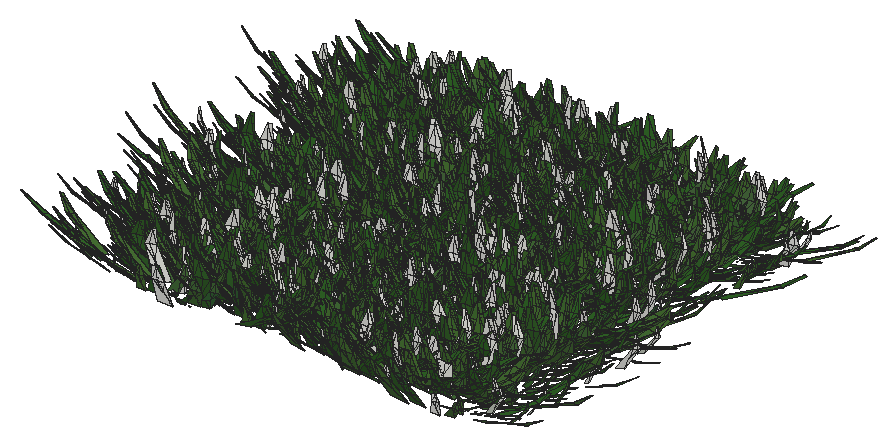
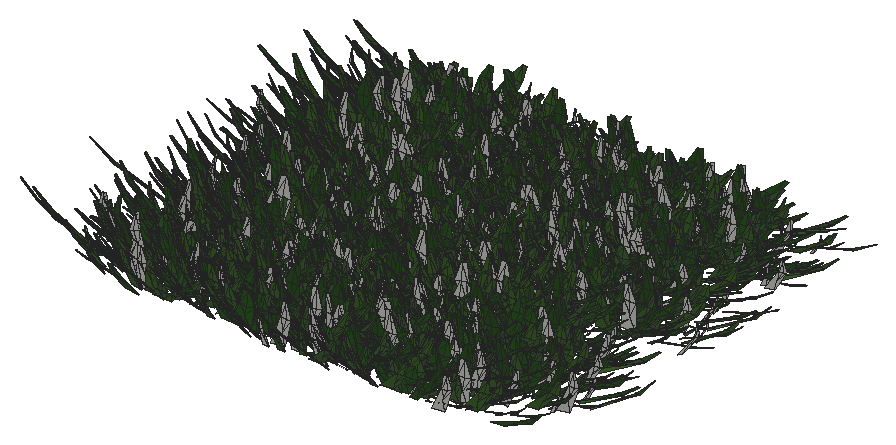
# SketchUp Ruby script. Lengths in inches.
U = 1.inch
M = Sketchup.active_model
def pt(a) = Geom::Point3d.new(a.map { |v| v * U })
def face(e, loops, mat)
  f = e.add_face(loops[0].map { |a| pt(a) })
  loops[1..].each { |l| e.add_face(l.map { |a| pt(a) }).erase! }
  f.material = f.back_material = mat if mat
  f
end
# faces: each face lists its corners as indices into pts; further lists are holes
def faces(e, pts, list, mat = nil) = list.each { |f| face(e, (f[0].is_a?(Array) ? f : [f]).map { |l| l.map { |i| pts[i] } }, mat) }
# xy, xz, yz: faces in a plane at the given z, y or x. An outline is a flat list of corners, or four numbers for a rectangle; further outlines are holes
def ring(l) = l.size == 4 ? [[l[0], l[1]], [l[2], l[1]], [l[2], l[3]], [l[0], l[3]]] : l.each_slice(2).to_a
def flat(e, list, mat, &to3) = list.each { |f| face(e, (f[0].is_a?(Array) ? f : [f]).map { |l| ring(l).map { |u, v| to3.(u, v) } }, mat) }
def xy(e, z, list, mat = nil) = flat(e, list, mat) { |x, y| [x, y, z] }
def xz(e, y, list, mat = nil) = flat(e, list, mat) { |x, z| [x, y, z] }
def yz(e, x, list, mat = nil) = flat(e, list, mat) { |y, z| [x, y, z] }
def lines(e, pts, list) = list.each { |a, b| e.add_line(pt(pts[a]), pt(pts[b])) }
# prism: a flat outline (further loops are holes) pulled along v
def prism(e, loops, v, mat = nil)
  f = face(e, loops, mat); d = Geom::Vector3d.new(v.map { |x| x * U })
  f.pushpull(f.normal.samedirection?(d) ? d.length : -d.length)
end
def box(e, o, s, mat = nil) = prism(e, [[o, [o[0] + s[0], o[1], o[2]], [o[0] + s[0], o[1] + s[1], o[2]], [o[0], o[1] + s[1], o[2]]]], [0, 0, s[2]], mat)
def at(x, y, z, deg = 0) = Geom::Transformation.translation(pt([x, y, z])) * Geom::Transformation.rotation(ORIGIN, Z_AXIS, deg.degrees)
def axes(o, x, y, z) = Geom::Transformation.new([*x, 0, *y, 0, *z, 0, *pt(o).to_a, 1])
def part(name) = M.definitions.add(name)
# library, detail: a bought-in or finely detailed component or shape, given as its bounding box
def library(name, o, s) = part(name).tap { |d| box(d.entities, o, s) }
def detail(e, o, s) = box(e.add_group.entities, o, s)
def put(e, d, t, mat = nil) = e.add_instance(d, t).tap { |i| i.material = mat if mat }
def group(e, t, mat = nil) = e.add_group.tap { |g| g.transformation = t; g.material = mat if mat }.entities
root = M.entities
M.materials.add("Material10").color = [48, 100, 38]
M.materials.add("Material3").color = [68, 110, 58]
M.materials.add("Material4").color = [48, 90, 38]
M.materials.add("Material5").color = [68, 110, 48]
M.materials.add("Material6").color = [48, 90, 48]
M.materials.add("Material7").color = [58, 110, 58]
M.materials.add("Material8").color = [58, 90, 38]
M.materials.add("Material9").color = [68, 100, 58]
c1 = part("grass00")
p = [[-0.6875,0.15,0],[-0.56,0.08,5.52],[-0.04,0.03,2.76],[0.48,-0.02,0],[0.35,-0.02,5.52],[-0.1,-0.14,5.52],
  [-0.12,0.65,8.37],[-0.42,0.65,8.37]]
faces(c1.entities,p,[[0,1,2,3],[3,2,4],[1,5,2],[5,4,2],[1,6,5],[4,5,6],[7,6,1]])
c2 = part("Group16\#1")
put(c2.entities,c1,axes([1.44,-0.61,-0.01],[0.05352,0.12609,0],[-0.10704,0.04543,0.07239],[0.06664,-0.02828,0.11628]),"Material6")
put(c2.entities,c1,axes([0.76,-0.15,-0.01],[0.04676,0.24062,0],[-0.23162,0.04501,0.06642],[0.0652,-0.01267,0.23595]),"Material3")
put(c2.entities,c1,axes([0.79,0.01,-0.01],[-0.00606,0.34651,0],[-0.34381,-0.00602,0.0432],[0.04319,0.00076,0.34386]))
put(c2.entities,c1,axes([1,0.23,-0.01],[-0.07192,0.31144,0],[-0.28722,-0.06632,0.1236],[0.12043,0.02781,0.29478]),"Material5")
put(c2.entities,c1,axes([1.66,0.77,-0.01],[-0.13828,0.29651,0],[-0.21551,-0.1005,0.22471],[0.20365,0.09498,0.23779]),"Material10")
put(c2.entities,c1,axes([0.6875,0.52,-0.01],[-0.18126,0.24051,0],[-0.22746,-0.17142,0.09788],[0.07817,0.05891,0.28481]),"Material5")
put(c2.entities,c1,axes([0.68,0.78,-0.01],[-0.215,0.18688,0],[-0.12385,-0.14248,0.21334],[0.13995,0.16101,0.18878]),"Material3")
put(c2.entities,c1,axes([0.56,1,-0.01],[-0.13756,0.07624,0],[-0.06159,-0.11112,0.0927],[0.04494,0.08108,0.12705]),"Material5")
put(c2.entities,c1,axes([0.2,0.64,-0.01],[-0.23729,0.07254,0],[-0.05711,-0.18681,0.153],[0.04473,0.14632,0.19535]),"Material10")
put(c2.entities,c1,axes([0.0625,0.72,-0.01],[-0.28874,0.02525,0],[-0.02179,-0.24916,0.14647],[0.01276,0.14591,0.25012]),"Material3")
put(c2.entities,c1,axes([-0.08,0.62,-0.01],[-0.34089,-0.04187,0],[0.03255,-0.26504,0.216],[-0.02633,0.21439,0.26703]),"Material10")
put(c2.entities,c1,axes([-0.34,0.98,-0.01],[-0.14314,-0.0493,0],[0.04397,-0.12769,0.06843],[-0.02228,0.0647,0.13505]),"Material10")
put(c2.entities,c1,axes([-0.87,1.45,-0.01],[-0.23488,-0.14114,0],[0.13761,-0.22901,0.06087],[-0.03135,0.05217,0.26717]))
put(c2.entities,c1,axes([-0.72,0.77,-0.01],[-0.14208,-0.13251,0],[0.07209,-0.0773,0.16301],[-0.11118,0.11922,0.1057]),"Material10")
put(c2.entities,c1,axes([-0.62,0.43,-0.01],[-0.14845,-0.21203,0],[0.18654,-0.13061,0.12304],[-0.10079,0.07057,0.22772]),"Material3")
put(c2.entities,c1,axes([-0.68,0.29,-0.01],[-0.13639,-0.32136,0],[0.31723,-0.13464,0.05579],[-0.05136,0.0218,0.34462]),"Material4")
put(c2.entities,c1,axes([-0.64,0.125,-0.01],[-0.0458,-0.23569,0],[0.22124,-0.043,0.08276],[-0.08124,0.01579,0.22538]),"Material7")
put(c2.entities,c1,axes([-1.6,-0.03,-0.01],[0.00576,-0.32897,0],[0.27526,0.00482,0.18018],[-0.18015,-0.00315,0.2753]),"Material5")
put(c2.entities,c1,axes([-1.36,-0.31,-0.01],[0.05718,-0.24765,0],[0.18172,0.04196,0.17267],[-0.16825,-0.03885,0.1865]),"Material10")
put(c2.entities,c1,axes([-1.54,-0.72,-0.01],[0.06537,-0.14017,0],[0.13555,0.06321,0.03939],[-0.0357,-0.01665,0.14956]))
put(c2.entities,c1,axes([-1.19,-0.9,-0.01],[0.09597,-0.12735,0],[0.11214,0.08451,0.07557],[-0.06035,-0.04548,0.14042]),"Material9")
put(c2.entities,c1,axes([-0.47,-0.54,-0.01],[0.11588,-0.10072,0],[0.0618,0.0711,0.12124],[-0.07953,-0.0915,0.0942]))
put(c2.entities,c1,axes([-0.47,-0.84,-0.01],[0.11927,-0.0661,0],[0.06603,0.11913,0.00646],[-0.00313,-0.00565,0.13621]),"Material5")
put(c2.entities,c1,axes([-0.38,-1.24,-0.01],[0.28037,-0.08571,0],[0.0618,0.20215,0.20315],[-0.05939,-0.19428,0.21139]),"Material9")
put(c2.entities,c1,axes([-0.06,-0.66,-0.01],[0.22719,-0.01987,0],[0.01247,0.14255,0.17758],[-0.01547,-0.17691,0.1431]),"Material8")
put(c2.entities,c1,axes([0.11,-0.89,-0.01],[0.14882,0.01828,0],[-0.01058,0.08611,0.12229],[0.01491,-0.12138,0.08676]),"Material6")
put(c2.entities,c1,axes([0.25,-0.72,-0.01],[0.20481,0.07053,0],[-0.06206,0.18022,0.10291],[0.03351,-0.0973,0.1906]),"Material6")
put(c2.entities,c1,axes([0.85,-1.42,-0.01],[0.16481,0.09904,0],[-0.09472,0.15762,0.05616],[0.02893,-0.04814,0.18389]),"Material5")
put(c2.entities,c1,axes([1.01,-1.09,-0.01],[0.21858,0.20385,0],[-0.17495,0.1876,0.15339],[0.10462,-0.11218,0.25652]),"Material10")
put(c2.entities,c1,axes([1.01,-0.71,-0.01],[0.08733,0.12473,0],[-0.06445,0.04512,0.13037],[0.1068,-0.07477,0.07867]),"Material6")
c3 = part("Group15\#1")
put(c3.entities,c2,at(0,0,0))
c4 = part("3darcstudiotree_grass00\#1")
put(c4.entities,c3,at(0,0,0))
put(root,c4,axes([159.13,10.51,7.6],[2.53298,-0.99579,0],[3.28482,0.52222,-0.04064],[0.20675,0.03287,1.46692]))
put(root,c4,axes([159.22,37.4375,7.6],[2.73989,-0.60489,0],[2.55091,0.72216,-0.01409],[0.06366,0.01802,1.64399]))
put(root,c4,axes([159.47,17.03,7.6],[2.49365,-0.78367,0],[3.24543,0.64544,-0.01848],[0.08233,0.01637,1.47553]))
put(root,c4,axes([158.3,36.26,7.6],[4.4609,0.40125,0],[-1.29285,0.89834,-0.01256],[-0.03244,0.02254,1.82155]))
put(root,c4,axes([158.47,24.0625,7.6],[2.4643,0.83625,0],[-3.57537,0.6585,-0.0323],[-0.14016,0.02581,1.496]))
put(root,c4,axes([159.16,32.27,7.6],[-1.53289,0.94847,0],[-3.89243,-0.39318,-0.02451],[-0.14378,-0.01452,1.66036]))
put(root,c4,axes([158.6,11.21,7.6],[3.75653,0.68918,0],[-2.16074,0.73611,-0.01519],[-0.05314,0.0181,1.34969]))
put(root,c4,axes([159.65,8.5625,7.6],[-1.332,1.0855,0],[-3.68359,-0.2825,-0.03727],[-0.23368,-0.01792,1.57911]))
put(root,c4,axes([158.96,20.36,7.6],[4.4023,0.31445,0],[-1.15221,1.00818,-0.01128],[-0.01903,0.01665,1.61003]))
put(root,c4,axes([159.3125,22.22,7.6],[4.69374,-0.30667,0],[0.9938,0.95067,-0.02428],[0.04983,0.04767,1.99391]))
put(root,c4,axes([159.65,34.32,7.6],[3.84654,0.1622,0],[-0.71389,1.05813,-0.03005],[-0.02875,0.04262,1.54341]))
put(root,c4,axes([160.2,5.28,7.6],[3.63097,-0.44195,0],[1.99155,1.02264,-0.02466],[0.05688,0.02921,1.49812]))
put(root,c4,axes([160.53,29.87,7.6],[-0.92615,0.92755,0],[-3.93926,-0.24583,-0.00012],[-0.00062,-0.00004,1.39497]))
put(root,c4,axes([160.89,40.6,7.6],[-1.66158,1.03755,0],[-3.61607,-0.36193,-0.01826],[-0.10251,-0.01026,1.47196]))
put(root,c4,axes([161.29,14.89,7.6],[3.53421,-0.66797,0],[2.63257,0.87056,-0.04167],[0.17144,0.05669,1.86151]))
put(root,c4,axes([162.89,12.95,7.6],[-3.75679,-0.65225,0],[2.19929,-0.79171,-0.00375],[0.0162,-0.00583,1.82358]))
put(root,c4,axes([162.96,8.51,7.6],[-3.06353,-0.57111,0],[2.62826,-0.88115,-0.00029],[0.00107,-0.00036,1.69542]))
put(root,c4,axes([161.18,31.73,7.6],[4.12285,0.65297,0],[-2.36966,0.93513,-0.03414],[-0.094,0.03709,1.42377]))
put(root,c4,axes([163.05,18.05,7.6],[-4.09682,0.49001,0],[-2.11354,-1.10442,-0.05113],[-0.09658,-0.05047,1.33965]))
put(root,c4,axes([163.35,33.23,7.6],[3.22149,-0.77184,0],[3.4883,0.90996,-0.03986],[0.14566,0.038,1.66404]))
put(root,c4,axes([163.88,5.03,7.6],[-3.99831,0.66373,0],[-2.79382,-1.05187,-0.05111],[-0.13772,-0.05185,1.53759]))
put(root,c4,axes([163.84,23.63,7.6],[-2.34879,0.82115,0],[-3.6953,-0.66061,-0.05929],[-0.24052,-0.043,1.41608]))
put(root,c4,axes([162.93,11.58,7.6],[2.86716,0.8976,0],[-2.85293,0.56956,-0.01421],[-0.0686,0.0137,1.40932]))
put(root,c4,axes([164.88,34.3,7.6],[-0.2584,-1.18473,0],[3.63618,-0.04957,-0.01049],[0.06761,-0.00092,1.4693]))
put(root,c4,axes([165.875,35.68,7.6],[-2.94405,-0.59903,0],[3.18153,-0.97726,-0.04334],[0.11663,-0.03583,1.34295]))
put(root,c4,axes([165.14,31.64,7.6],[2.52087,-0.77867,0],[3.74489,0.75773,-0.0352],[0.16916,0.03423,1.86157]))
put(root,c4,axes([166.21,29.5625,7.6],[-4.25461,-0.72001,0],[2.67413,-0.98761,-0.04034],[0.12328,-0.04553,1.62559]))
put(root,c4,axes([163.93,16.3,7.6],[4.6579,0.46394,0],[-1.71341,1.07515,-0.01606],[-0.03179,0.01995,1.54782]))
put(root,c4,axes([164.26,28.29,7.6],[1.00242,0.87576,0],[-4.78791,0.34253,-0.02742],[-0.16399,0.01173,1.93645]))
put(root,c4,axes([164.54,21.99,7.6],[-0.10924,0.93543,0],[-4.47278,-0.03265,-0.00454],[-0.02701,-0.0002,1.66362]))
put(root,c4,axes([166.71,20.63,7.6],[-1.41075,-1.20737,0],[3.77402,-0.27561,-0.03009],[0.20256,-0.01479,1.72353]))
put(root,c4,axes([165.51,42.17,7.6],[4.18656,0.30844,0],[-1.02812,0.87218,-0.026],[-0.05159,0.04376,1.59572]))
put(root,c4,axes([167.1875,39.94,7.6],[1.76759,-1.11088,0],[4.77436,0.4748,-0.04298],[0.2101,0.02089,1.68954]))
put(root,c4,axes([165.72,38.26,7.6],[4.47643,0.35496,0],[-1.36564,1.07638,-0.00141],[-0.00295,0.00232,1.95289]))
put(root,c4,axes([166.25,7.31,7.6],[0.44827,0.96887,0],[-3.98401,0.1152,-0.04522],[-0.2884,0.00834,1.60941]))
put(root,c4,axes([166.69,10.33,7.6],[-3.25483,0.8021,0],[-3.45367,-0.87591,-0.01243],[-0.05011,-0.01271,1.76595]))
put(root,c4,axes([166.71,36.98,7.6],[4.42338,-0.02191,0],[0.0799,1.00813,-0.01855],[0.00282,0.03561,1.93628]))
put(root,c4,axes([166.8,14.59,7.6],[1.52901,1.13008,0],[-3.97535,0.33617,-0.04556],[-0.25323,0.02141,1.53888]))
put(root,c4,axes([167.35,18.53,7.6],[4.69014,-0.44413,0],[1.55704,1.02768,-0.01068],[0.01805,0.01192,1.31138]))
put(root,c4,axes([167.31,27.18,7.6],[3.67709,0.37589,0],[-1.7272,1.05602,-0.03911],[-0.07805,0.04772,1.50402]))
put(root,c4,axes([169.42,21.05,7.6],[-2.16175,-1.00389,0],[3.8462,-0.51764,-0.02018],[0.12706,-0.0171,1.95264]))
put(root,c4,axes([169.36,31.17,7.6],[-2.62411,-0.67542,0],[2.85989,-0.69444,-0.02073],[0.09247,-0.02245,1.5494]))
put(root,c4,axes([167.22,25.11,7.6],[2.20682,1.15051,0],[-3.88825,0.46614,-0.00104],[-0.00548,0.00066,1.58037]))
put(root,c4,axes([169.95,29.43,7.6],[-3.73719,-0.68313,0],[2.19401,-0.75016,-0.03203],[0.15881,-0.0543,1.95145]))
put(root,c4,axes([169.06,5.71,7.6],[3.66888,-0.3039,0],[1.21402,0.91602,-0.03222],[0.07511,0.05667,1.78787]))
put(root,c4,axes([169.76,41.57,7.6],[2.44539,-0.83578,0],[3.06971,0.56135,-0.02877],[0.14565,0.02664,1.49076]))
put(root,c4,axes([171.36,26.94,7.6],[-2.07648,-1.05782,0],[4.05072,-0.49696,-0.01008],[0.05023,-0.00616,1.566]))
put(root,c4,axes([169.62,8.06,7.6],[0.11038,0.92839,0],[-4.43569,0.03296,-0.05613],[-0.30865,0.00229,1.5259]))
put(root,c4,axes([170.4,23.125,7.6],[3.30121,-0.61217,0],[2.52484,0.85098,-0.02804],[0.09819,0.03309,1.55696]))
put(root,c4,axes([169.56,7.46,7.6],[2.77049,0.67206,0],[-2.57835,0.66431,-0.00683],[-0.0359,0.00925,1.74693]))
put(root,c4,axes([171.22,38.9375,7.6],[-4.82674,0.25422,0],[-0.88565,-1.05095,-0.00142],[-0.00177,-0.0021,1.63114]))
put(root,c4,axes([171.51,24.73,7.6],[-4.23216,-0.4101,0],[1.59131,-1.02639,-0.05586],[0.14093,-0.0909,1.92103]))
put(root,c4,axes([171.66,13.95,7.6],[0.04875,-0.97285,0],[3.90965,0.01225,-0.00992],[0.05364,0.00017,1.32167]))
put(root,c4,axes([171.35,40.41,7.6],[-4.10192,0.74973,0],[-2.75988,-0.94373,-0.03994],[-0.15914,-0.05442,1.97331]))
put(root,c4,axes([170.21,35.1875,7.6],[5.03069,0.15304,0],[-0.59852,1.22962,-0.0359],[-0.02633,0.0541,1.88046]))
put(root,c4,axes([171.68,32.1875,7.6],[1.61139,-0.92057,0],[3.30633,0.36172,-0.00213],[0.01129,0.00123,1.30651]))
put(root,c4,axes([172.91,9.63,7.6],[-2.89418,-0.78817,0],[3.81113,-0.87466,-0.02326],[0.09657,-0.02216,1.82249]))
put(root,c4,axes([172.31,11.86,7.6],[1.38566,-1.0009,0],[3.42279,0.29616,-0.00044],[0.00245,0.00021,1.32507]))
put(root,c4,axes([172.875,18.86,7.6],[-4.53149,-0.15613,0],[0.63638,-1.15439,-0.00876],[0.00543,-0.00985,1.32289]))
put(root,c4,axes([171.83,34.23,7.6],[-3.16538,1.0009,0],[-3.18179,-0.62891,-0.0043],[-0.02493,-0.00493,1.8735]))
put(root,c4,axes([170.84,28.53,7.6],[2.46284,0.96083,0],[-4.30352,0.68944,-0.02786],[-0.14516,0.02326,1.9768]))
put(root,c4,axes([171.89,12.7,7.6],[3.73009,0.22757,0],[-0.89297,0.9148,-0.01459],[-0.0258,0.02643,1.75568]))
put(root,c4,axes([172.13,37.66,7.6],[5.05197,-0.08472,0],[0.33414,1.24538,-0.00473],[0.00152,0.00566,1.49489]))
put(root,c4,axes([172.04,16.05,7.6],[3.94341,0.43089,0],[-1.69112,0.9673,-0.01451],[-0.03524,0.02016,1.59989]))
put(root,c4,axes([173.25,17.83,7.6],[-1.02018,1.09305,0],[-3.99403,-0.23299,-0.02125],[-0.10851,-0.00633,1.34411]))
put(root,c4,axes([173.11,21.67,7.6],[1.6819,1.04129,0],[-4.31148,0.43525,-0.05886],[-0.25156,0.0254,1.33951]))
put(root,c4,axes([175.58,17.4375,7.6],[-2.51512,-0.77135,0],[3.2397,-0.66023,-0.00371],[0.01648,-0.00336,1.4993]))
put(root,c4,axes([175.5,42,7.6],[-2.73008,-0.65952,0],[3.11842,-0.80679,-0.03177],[0.14282,-0.03695,1.8145]))
put(root,c4,axes([175.29,21.77,7.6],[-3.14493,1.01166,0],[-3.08712,-0.59981,-0.03149],[-0.13615,-0.02645,1.33797]))
put(root,c4,axes([175.24,15.97,7.6],[-3.00004,0.96775,0],[-4.04392,-0.78352,-0.03455],[-0.13505,-0.02617,1.58129]))
put(root,c4,axes([176.8125,35.56,7.6],[-3.06002,-0.4895,0],[1.9457,-0.7602,-0.02395],[0.07981,-0.03118,1.39534]))
put(root,c4,axes([175.51,9.49,7.6],[4.73916,-0.2961,0],[1.22977,1.23018,-0.03338],[0.03516,0.03517,1.37691]))
put(root,c4,axes([175.81,27.67,7.6],[3.7155,-0.16397,0],[0.83101,1.17689,-0.03701],[0.04274,0.06052,1.98432]))
put(root,c4,axes([175.75,33.74,7.6],[1.11685,0.86772,0],[-3.58583,0.28846,-0.0339],[-0.24805,0.01995,1.80984]))
put(root,c4,axes([176.24,14.33,7.6],[3.47383,0.27183,0],[-1.15707,0.92418,-0.01935],[-0.04591,0.03667,1.92273]))
put(root,c4,axes([176.59,26.11,7.6],[3.76768,-0.14266,0],[0.7468,1.23267,-0.05863],[0.04677,0.07719,1.66018]))
put(root,c4,axes([177.47,40.64,7.6],[-2.77251,0.84183,0],[-3.16826,-0.65216,-0.04557],[-0.25419,-0.05232,1.85346]))
put(root,c4,axes([178.3,8.63,7.6],[-4.19889,-0.35497,0],[1.51882,-1.12287,-0.06149],[0.11991,-0.08865,1.80385]))
put(root,c4,axes([178.42,25.61,7.6],[-2.26034,-0.95612,0],[4.04504,-0.59768,-0.04139],[0.22409,-0.03311,1.84708]))
put(root,c4,axes([176.44,32.35,7.6],[2.33279,0.76327,0],[-3.38254,0.64613,-0.0123],[-0.05875,0.01122,1.59876]))
put(root,c4,axes([178.72,36.75,7.6],[-4.70227,-0.09202,0],[0.37427,-1.19528,-0.05117],[0.02052,-0.06554,1.54048]))
put(root,c4,axes([177.22,5.27,7.6],[4.48386,0.0868,0],[-0.3465,1.11875,-0.0417],[-0.02197,0.07094,1.91485]))
put(root,c4,axes([178.7,23.11,7.6],[-4.35252,0.40027,0],[-1.39021,-0.94482,-0.04924],[-0.13398,-0.09105,1.98345]))
put(root,c4,axes([177.3125,31.51,7.6],[5.08464,-0.02369,0],[0.09161,1.22889,-0.03615],[0.00341,0.04568,1.55355]))
put(root,c4,axes([177.14,6.88,7.6],[3.96051,0.53501,0],[-2.37184,1.09738,-0.05913],[-0.12576,0.05819,1.39517]))
put(root,c4,axes([178.69,11.46,7.6],[-3.78367,0.13136,0],[-0.66281,-1.19321,-0.02154],[-0.01411,-0.0254,1.4342]))
put(root,c4,axes([178.02,12.61,7.6],[1.46709,1.05523,0],[-3.46881,0.30142,-0.01128],[-0.08445,0.00734,1.81963]))
put(root,c4,axes([178.64,19.5625,7.6],[-0.91674,0.93893,0],[-3.90242,-0.23814,-0.03757],[-0.1913,-0.01167,1.3158]))
put(root,c4,axes([179.47,21.13,7.6],[3.37683,-0.41478,0],[2.02863,1.03221,-0.05746],[0.17419,0.08863,1.97658]))
put(root,c4,axes([179.35,30.17,7.6],[1.70448,0.82052,0],[-3.56359,0.46267,-0.04821],[-0.23323,0.03028,1.36797]))
put(root,c4,axes([179.5,38.89,7.6],[0.92537,0.88194,0],[-4.41154,0.2893,-0.05161],[-0.26626,0.01746,1.52021]))
put(root,c4,axes([181.91,24.97,7.6],[-4.05837,-0.6928,0],[2.05635,-0.75288,-0.01838],[0.08227,-0.03012,1.80866]))
put(root,c4,axes([181.93,36.15,7.6],[0.10765,-0.97031,0],[3.90714,0.02709,-0.00183],[0.01108,0.00008,1.48199]))
put(root,c4,axes([181.59,11.97,7.6],[2.38443,-0.79485,0],[3.89504,0.73029,-0.03529],[0.12587,0.0236,1.35654]))
put(root,c4,axes([182.61,20.68,7.6],[-4.4757,-0.23245,0],[1.02085,-1.22848,-0.02537],[0.03005,-0.03616,1.82613]))
put(root,c4,axes([182.24,28.28,7.6],[-4.25208,0.35979,0],[-1.19702,-0.88418,-0.02484],[-0.06716,-0.04961,1.96802]))
put(root,c4,axes([182.55,14.57,7.6],[-4.39783,0.19091,0],[-0.81712,-1.17645,-0.05401],[-0.04088,-0.05885,1.3206]))
put(root,c4,axes([181.94,17.9,7.6],[-2.10693,0.77136,0],[-3.00017,-0.51217,-0.01899],[-0.12155,-0.02075,1.75992]))
put(root,c4,axes([181.21,5.08,7.6],[-0.15623,0.94532,0],[-4.49196,-0.0464,-0.00296],[-0.0156,-0.00016,1.47961]))
put(root,c4,axes([181.5,21.61,7.6],[-0.40598,1.27803,0],[-4.68179,-0.09295,-0.01448],[-0.07168,-0.00142,1.45727]))
put(root,c4,axes([181.73,41.625,7.6],[4.58397,0.20442,0],[-0.68449,0.9593,-0.04495],[-0.06411,0.08985,1.97854]))
put(root,c4,axes([184.01,23.1875,7.6],[-0.75592,-0.93689,0],[4.57802,-0.23086,-0.04603],[0.25634,-0.01293,1.65834]))
put(root,c4,axes([182.49,6.5,7.6],[4.03398,0.31007,0],[-1.40845,1.14523,-0.02064],[-0.02977,0.02421,1.46981]))
put(root,c4,axes([183.96,32.33,7.6],[-4.15465,0.6663,0],[-2.35272,-0.91688,-0.01729],[-0.05585,-0.02177,1.62898]))
put(root,c4,axes([184.66,12.53,7.6],[-3.83717,-0.19208,0],[0.9693,-1.21021,-0.02406],[0.02351,-0.02935,1.53532]))
put(root,c4,axes([184.96,37.23,7.6],[-4.91779,-0.19601,0],[0.6703,-1.05111,-0.05098],[0.05043,-0.07908,1.67187]))
put(root,c4,axes([183.38,29.94,7.6],[4.59957,-0.09357,0],[0.3643,1.11918,-0.01977],[0.00913,0.02806,1.59866]))
put(root,c4,axes([184.77,31.05,7.6],[-4.94513,0.23867,0],[-0.82278,-1.06546,-0.00152],[-0.0015,-0.00195,1.41339]))
put(root,c4,axes([183.61,26.07,7.6],[-1.34706,1.11667,0],[-4.07742,-0.30742,-0.01363],[-0.0693,-0.00522,1.41312]))
put(root,c4,axes([184.35,8.62,7.6],[-2.30928,0.69091,0],[-3.20293,-0.66909,-0.03387],[-0.15372,-0.03211,1.54303]))
put(root,c4,axes([184.18,10.125,7.6],[3.65365,-0.40447,0],[2.03299,1.14777,-0.04981],[0.11291,0.06375,1.75709]))
put(root,c4,axes([183.83,34.23,7.6],[2.59051,0.81942,0],[-3.35986,0.66386,-0.02315],[-0.11156,0.02204,1.64391]))
put(root,c4,axes([183.7,40.33,7.6],[2.96025,0.64544,0],[-3.39185,0.97228,-0.01764],[-0.06278,0.018,1.74631]))
put(root,c4,axes([185.12,18.98,7.6],[3.11892,-0.94287,0],[3.04529,0.6296,-0.04304],[0.23637,0.04887,1.76026]))
put(root,c4,axes([184.52,15.56,7.6],[0.28426,1.04534,0],[-4.32493,0.07351,-0.02807],[-0.13623,0.00232,1.3177]))
put(root,c4,axes([187.37,5.76,7.6],[-2.81125,-0.60832,0],[3.02098,-0.87256,-0.00422],[0.01275,-0.00368,1.33295]))
put(root,c4,axes([185.49,38.68,7.6],[3.79286,0.40503,0],[-1.76539,1.03325,-0.00364],[-0.00998,0.00584,1.96053]))
put(root,c4,axes([188.6,37.48,7.6],[-2.87569,-1.00726,0],[3.7505,-0.66922,-0.01802],[0.06852,-0.01223,1.345]))
put(root,c4,axes([188.0625,31.4,7.6],[-3.91989,0.02908,0],[-0.12642,-1.06499,-0.02538],[-0.00493,-0.04149,1.74242]))
put(root,c4,axes([187.26,15.99,7.6],[-2.30919,0.93176,0],[-3.9041,-0.60472,-0.01218],[-0.05759,-0.00892,1.59607]))
put(root,c4,axes([188.03,11.78,7.6],[3.80375,-0.52233,0],[2.25643,1.02699,-0.02691],[0.07906,0.03598,1.78778]))
put(root,c4,axes([189.43,6.9,7.6],[-1.71233,-0.84239,0],[3.99342,-0.50734,-0.00876],[0.04062,-0.00516,1.45672]))
put(root,c4,axes([189.68,17.46,7.6],[-3.48158,-0.93813,0],[3.46536,-0.80378,-0.01209],[0.04881,-0.01132,1.62724]))
put(root,c4,axes([189.75,20.35,7.6],[-2.81575,-0.88554,0],[3.65217,-0.7258,-0.01168],[0.04216,-0.00838,1.34439]))
put(root,c4,axes([187.9,28.01,7.6],[-0.1762,1.09115,0],[-4.68185,-0.04725,-0.04298],[-0.27686,-0.00279,1.88799]))
put(root,c4,axes([189.81,23.39,7.6],[-3.80607,-0.23651,0],[1.18989,-1.19677,-0.01735],[0.0231,-0.02323,1.70162]))
put(root,c4,axes([189.71,25.55,7.6],[-3.60582,-0.24196,0],[1.04886,-0.97693,-0.03217],[0.06139,-0.05718,1.86146]))
put(root,c4,axes([187.77,10.43,7.6],[2.28978,0.96186,0],[-3.76338,0.55994,-0.00188],[-0.01111,0.00165,1.87843]))
put(root,c4,axes([188.21,26.71,7.6],[2.13866,0.74246,0],[-3.14038,0.56537,-0.02117],[-0.12042,0.02168,1.69559]))
put(root,c4,axes([188.95,18.78,7.6],[-2.16053,0.9205,0],[-4.3515,-0.63835,-0.01374],[-0.05636,-0.00827,1.50009]))
put(root,c4,axes([188.56,4.26,7.6],[0.82896,1.15167,0],[-5.08245,0.22864,-0.03105],[-0.14233,0.0064,1.50318]))
put(root,c4,axes([188.76,29.82,7.6],[4.96916,0.09392,0],[-0.36542,1.20834,-0.04634],[-0.02294,0.07584,1.98901]))
put(root,c4,axes([188.91,36.16,7.6],[1.48031,1.01744,0],[-4.79783,0.43628,-0.0524],[-0.2112,0.01921,1.36852]))
put(root,c4,axes([190.98,39.05,7.6],[-4.63446,-0.46393,0],[1.56749,-0.97866,-0.04264],[0.10164,-0.06346,1.69007]))
put(root,c4,axes([189.91,40.74,7.6],[3.16295,-0.50135,0],[2.10496,0.83,-0.03299],[0.1278,0.05039,1.77748]))
put(root,c4,axes([190.54,13.5,7.6],[-3.25579,0.4273,0],[-2.23495,-1.06431,-0.02543],[-0.07509,-0.03576,1.9093]))
put(root,c4,axes([189.76,41.75,7.6],[2.11626,0.74991,0],[-2.96839,0.52355,-0.03223],[-0.15972,0.02817,1.37708]))
put(root,c4,axes([190.16,14.89,7.6],[2.21507,0.97624,0],[-3.15725,0.44774,-0.03898],[-0.29704,0.04212,1.98748]))
put(root,c4,axes([190.56,34.29,7.6],[2.51481,0.74573,0],[-2.81558,0.59343,-0.04117],[-0.21226,0.04474,1.55213]))
put(root,c4,axes([190.53,8.4375,7.6],[0.22886,1.14034,0],[-4.67986,0.0587,-0.03261],[-0.20676,0.00259,1.85888]))
put(root,c4,axes([190.37,22.4,7.6],[1.19223,1.00137,0],[-3.72637,0.27729,-0.00785],[-0.05882,0.00438,1.89978]))
put(root,c4,axes([190.61,32.97,7.6],[2.95745,0.80625,0],[-2.67106,0.61236,-0.03804],[-0.21785,0.04994,1.7602]))
